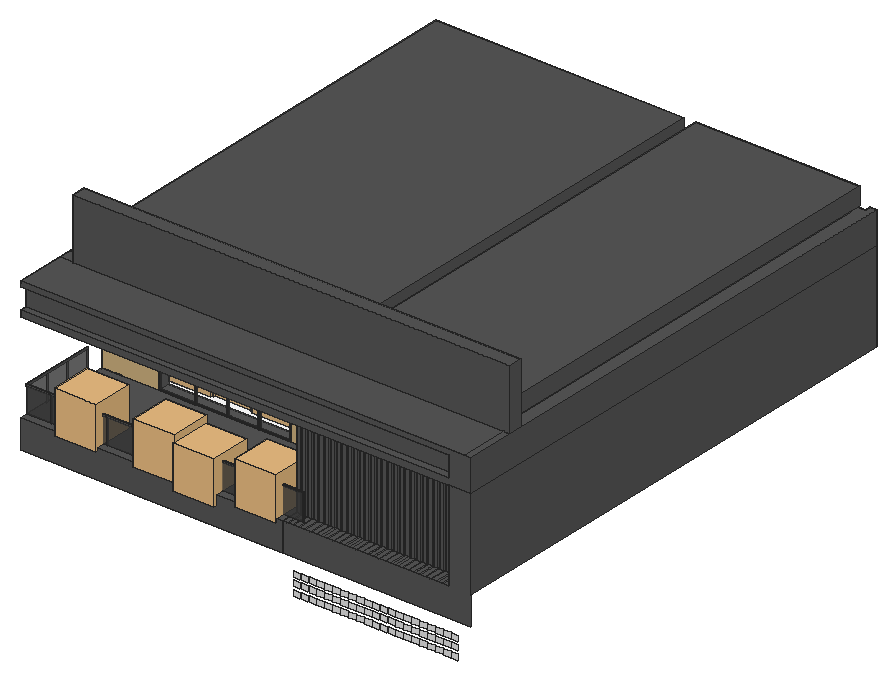
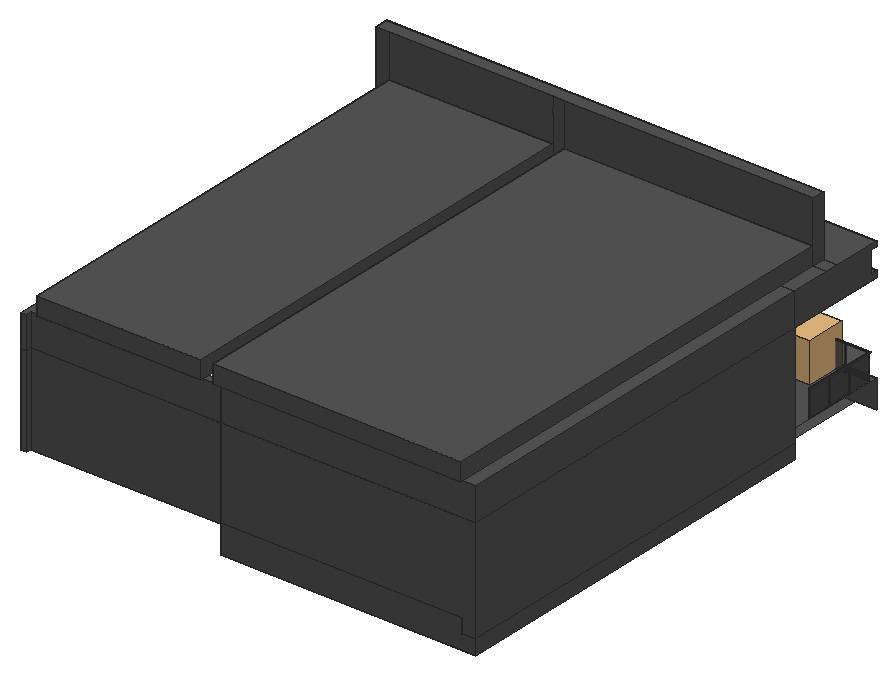
# SketchUp Ruby script. Lengths in inches.
U = 1.inch
M = Sketchup.active_model
def pt(a) = Geom::Point3d.new(a.map { |v| v * U })
def face(e, loops, mat)
  f = e.add_face(loops[0].map { |a| pt(a) })
  loops[1..].each { |l| e.add_face(l.map { |a| pt(a) }).erase! }
  f.material = f.back_material = mat if mat
  f
end
# faces: each face lists its corners as indices into pts; further lists are holes
def faces(e, pts, list, mat = nil) = list.each { |f| face(e, (f[0].is_a?(Array) ? f : [f]).map { |l| l.map { |i| pts[i] } }, mat) }
# xy, xz, yz: faces in a plane at the given z, y or x. An outline is a flat list of corners, or four numbers for a rectangle; further outlines are holes
def ring(l) = l.size == 4 ? [[l[0], l[1]], [l[2], l[1]], [l[2], l[3]], [l[0], l[3]]] : l.each_slice(2).to_a
def flat(e, list, mat, &to3) = list.each { |f| face(e, (f[0].is_a?(Array) ? f : [f]).map { |l| ring(l).map { |u, v| to3.(u, v) } }, mat) }
def xy(e, z, list, mat = nil) = flat(e, list, mat) { |x, y| [x, y, z] }
def xz(e, y, list, mat = nil) = flat(e, list, mat) { |x, z| [x, y, z] }
def yz(e, x, list, mat = nil) = flat(e, list, mat) { |y, z| [x, y, z] }
def lines(e, pts, list) = list.each { |a, b| e.add_line(pt(pts[a]), pt(pts[b])) }
# prism: a flat outline (further loops are holes) pulled along v
def prism(e, loops, v, mat = nil)
  f = face(e, loops, mat); d = Geom::Vector3d.new(v.map { |x| x * U })
  f.pushpull(f.normal.samedirection?(d) ? d.length : -d.length)
end
def box(e, o, s, mat = nil) = prism(e, [[o, [o[0] + s[0], o[1], o[2]], [o[0] + s[0], o[1] + s[1], o[2]], [o[0], o[1] + s[1], o[2]]]], [0, 0, s[2]], mat)
def at(x, y, z, deg = 0) = Geom::Transformation.translation(pt([x, y, z])) * Geom::Transformation.rotation(ORIGIN, Z_AXIS, deg.degrees)
def axes(o, x, y, z) = Geom::Transformation.new([*x, 0, *y, 0, *z, 0, *pt(o).to_a, 1])
def part(name) = M.definitions.add(name)
# library, detail: a bought-in or finely detailed component or shape, given as its bounding box
def library(name, o, s) = part(name).tap { |d| box(d.entities, o, s) }
def detail(e, o, s) = box(e.add_group.entities, o, s)
def put(e, d, t, mat = nil) = e.add_instance(d, t).tap { |i| i.material = mat if mat }
def group(e, t, mat = nil) = e.add_group.tap { |g| g.transformation = t; g.material = mat if mat }.entities
root = M.entities
M.materials.add("Glazing").color = [128, 128, 128]
M.materials["Glazing"].alpha = 0.05
M.materials.add("Powdercoating").color = [41, 44, 40]
M.materials.add("[0135_DarkGray]").color = [81, 81, 81]
M.materials.add("[Color M06]").color = [86, 86, 86]
M.materials.add("[Polished Concrete Old]").color = [229, 229, 229]
M.materials.add("[Translucent Glass Safety]").color = [204, 235, 244]
M.materials["[Translucent Glass Safety]"].alpha = 0.5
M.materials.add("[Translucent_Glass_Gray]").color = [63, 63, 63]
M.materials["[Translucent_Glass_Gray]"].alpha = 0.54
M.materials.add("[Wood Floor Light]").color = [204, 176, 127]
c1 = library("Pot+Plant",[-20.81,-17.08,-0.03],[39.86,39.43,41.33])
c2 = part("Group\#15")
xy(c2.entities,0,[[0,-55.94,0.71,45.94]])
xy(c2.entities,0.2,[[0,-55.94,0.47,45.94],[0.47,45.94,0.71,46.42]])
xy(c2.entities,2.36,[[0.47,-55.94,0.71,46.42]])
xz(c2.entities,-55.94,[[0,0,0.71,0,0.71,2.36,0.47,2.36,0.47,0.2,0,0.2]])
xz(c2.entities,45.94,[[0,0,0.71,0.2]])
xz(c2.entities,46.42,[[0.47,0.2,0.71,2.36]])
yz(c2.entities,0,[[-55.94,0,45.94,0.2]])
yz(c2.entities,0.47,[[-55.94,0.2,46.42,2.36]])
yz(c2.entities,0.71,[[-55.94,0,45.94,0,45.94,0.2,46.42,0.2,46.42,2.36,-55.94,2.36]])
c3 = part("Group\#7")
xy(c3.entities,0,[[0,-59.09,0.71,45.94]])
xy(c3.entities,0.2,[[0,-59.09,0.47,45.94],[0.47,45.94,0.71,46.42]])
xy(c3.entities,2.36,[[0.47,-59.09,0.71,46.42]])
xz(c3.entities,-59.09,[[0,0,0.71,0,0.71,2.36,0.47,2.36,0.47,0.2,0,0.2]])
xz(c3.entities,45.94,[[0,0,0.71,0.2]])
xz(c3.entities,46.42,[[0.47,0.2,0.71,2.36]])
yz(c3.entities,0,[[-59.09,0,45.94,0.2]])
yz(c3.entities,0.47,[[-59.09,0.2,46.42,2.36]])
yz(c3.entities,0.71,[[-59.09,0,45.94,0,45.94,0.2,46.42,0.2,46.42,2.36,-59.09,2.36]])
c4 = part("Group\#16")
prism(c4.entities,[[[0.47,-56.18,0.2],[0,-56.18,0.2],[0,-56.18,0],[0.71,-56.18,0],[0.71,-56.18,2.36],[0.47,-56.18,2.36]]],[0,28.68,0])
c5 = part("Group\#10")
box(c5.entities,[-0.73,0,0],[27.99,0.55,102.05])
c6 = part("Group\#18")
xy(c6.entities,0,[[0.47,-56.18,0.47,-55.47,0,-55.47,0,-28.21,1.18,-28.21,1.18,-56.18]])
xy(c6.entities,0.2,[[0.71,-56.18,1.18,-28.21],[0,-55.47,0.47,-28.21],[0.47,-28.21,0.71,-27.74]])
xy(c6.entities,2.36,[[0.47,-56.18,0.71,-27.74]])
xz(c6.entities,-56.18,[[0.47,0,1.18,0,1.18,0.2,0.71,0.2,0.71,2.36,0.47,2.36]])
xz(c6.entities,-55.47,[[0,0,0.47,0.2]])
xz(c6.entities,-28.21,[[0,0,1.18,0.2]])
xz(c6.entities,-27.74,[[0.47,0.2,0.71,2.36]])
yz(c6.entities,0,[[-55.47,0,-28.21,0.2]])
yz(c6.entities,0.47,[[-56.18,0,-55.47,0.2],[-56.18,0.2,-27.74,2.36]])
yz(c6.entities,0.71,[[-56.18,0.2,-27.74,2.36]])
yz(c6.entities,1.18,[[-56.18,0,-28.21,0.2]])
c7 = part("Group\#34")
xy(c7.entities,0,[[-20.45,0,7.76,1.22]])
xy(c7.entities,0.06,[[-20.39,0.06,7.7,1.22]])
xy(c7.entities,0.47,[[-19.98,0,7.28,0.06]])
xy(c7.entities,101.89,[[-19.98,0,7.28,0.06]])
xy(c7.entities,102.3,[[-20.39,0.06,7.7,1.22]])
xy(c7.entities,102.36,[[-20.45,0,7.76,1.22]])
xz(c7.entities,0,[[[-20.45,0,7.76,102.36],[-19.98,0.47,7.28,101.89]]])
xz(c7.entities,0.06,[[[-20.39,0.06,7.7,102.3],[-19.98,0.47,7.28,101.89]]])
xz(c7.entities,1.22,[[[-20.45,0,7.76,102.36],[-20.39,0.06,7.7,102.3]]])
yz(c7.entities,-20.45,[[0,0,1.22,102.36]])
yz(c7.entities,-20.39,[[0.06,0.06,1.22,102.3]])
yz(c7.entities,-19.98,[[0,0.47,0.06,101.89]])
yz(c7.entities,7.28,[[0,0.47,0.06,101.89]])
yz(c7.entities,7.7,[[0.06,0.06,1.22,102.3]])
yz(c7.entities,7.76,[[0,0,1.22,102.36]])
c8 = part("Group\#6")
put(c8.entities,c2,axes([27.97,0,7.875],[1,0,0],[0,0,-1],[0,1,0]),"Powdercoating")
put(c8.entities,c3,axes([0.71,0,6.8],[-1,0,0],[0,0,-0.97687],[0,1,0]),"Powdercoating")
put(c8.entities,c4,axes([-27.5,0,-38.07],[0,0,-1],[-1,0,0],[0,1,0]),"Powdercoating")
put(c8.entities,c5,at(1.12,0.35,-38.39),"Glazing")
put(c8.entities,c6,axes([-27.5,0,63.35],[0,0,1],[-1,0,0],[0,1,0]),"Powdercoating")
put(c8.entities,c7,at(20.6875,1.0625,-38.54),"Powdercoating")
c9 = part("Sliding door panels")
put(c9.entities,c8,at(-1.18,4.5,38.86))
g1 = group(c9.entities,at(84.74,4.5,38.86))
put(g1,c2,axes([-27.97,0,7.875],[-1,0,0],[0,0,-1],[0,1,0]),"Powdercoating")
put(g1,c3,axes([-0.71,0,6.8],[1,0,0],[0,0,-0.97687],[0,1,0]),"Powdercoating")
put(g1,c4,axes([27.5,0,-38.07],[0,0,-1],[1,0,0],[0,1,0]),"Powdercoating")
put(g1,c5,axes([-1.12,0.35,-38.39],[-1,0,0],[0,1,0],[0,0,1]),"Glazing")
put(g1,c6,axes([27.5,0,63.35],[0,0,1],[1,0,0],[0,1,0]),"Powdercoating")
put(g1,c7,axes([-20.6875,1.0625,-38.54],[-1,0,0],[0,1,0],[0,0,1]),"Powdercoating")
g2 = group(c9.entities,at(56.0625,4.5,38.86))
put(g2,c2,axes([-27.97,0,7.875],[-1,0,0],[0,0,-1],[0,1,0]),"Powdercoating")
put(g2,c4,axes([27.5,0,-38.07],[0,0,-1],[1,0,0],[0,1,0]),"Powdercoating")
put(g2,c5,axes([-1.12,0.35,-38.39],[-1,0,0],[0,1,0],[0,0,1]),"Glazing")
put(g2,c6,axes([27.5,0,63.35],[0,0,1],[1,0,0],[0,1,0]),"Powdercoating")
put(g2,c7,axes([-20.6875,1.0625,-38.54],[-1,0,0],[0,1,0],[0,0,1]),"Powdercoating")
g3 = group(g2,at(-0.71,0,6.8),"Powdercoating")
xy(g3,-45.34,[[0.47,0.2,0.71,2.36]])
xy(g3,-44.88,[[0,0,0.71,0.2]])
xy(g3,57.73,[[0,0,0.71,0,0.71,2.36,0.47,2.36,0.47,0.2,0,0.2]])
xz(g3,0,[[0,-44.88,0.71,57.73]])
xz(g3,0.2,[[0.47,-45.34,0.71,-44.88],[0,-44.88,0.47,57.73]])
xz(g3,2.36,[[0.47,-45.34,0.71,57.73]])
yz(g3,0,[[0,-44.88,0.2,57.73]])
yz(g3,0.47,[[0.2,-45.34,2.36,57.73]])
yz(g3,0.71,[[0.2,-45.34,2.36,-45.34,2.36,57.73,0,57.73,0,-44.88,0.2,-44.88]])
put(c9.entities,c8,axes([-33.94,4.5,38.86],[1.14218,0,0],[0,1,0],[0,0,1]))
c10 = part("sliding door")
put(c10.entities,c9,at(0,-4.5,-0.08))
c11 = part("Group\#81")
box(c11.entities,[0,0,0],[0.79,39.37,35.43],"[Translucent_Glass_Gray]")
c12 = part("Group\#82")
box(c12.entities,[0,0,0],[0.59,1.57,34.25])
c13 = part("Group\#85")
g4 = group(c13.entities,at(0.55,0.5,0))
put(g4,c11,axes([293.06,0,0],[0,0.84,0],[-0.92977,0,0],[0,0,1]),"[Translucent Glass Safety]")
g5 = group(g4,at(0,33.57,0),"[Translucent Glass Safety]")
box(g5,[0,0,0],[0.73,33.07,35.43],"[Translucent_Glass_Gray]")
put(g4,c11,axes([218.38,0,0],[0,0.84,0],[-0.92977,0,0],[0,0,1]),"[Translucent Glass Safety]")
put(g4,c11,axes([367.73,0,0],[0,0.84,0],[-0.92977,0,0],[0,0,1]),"[Translucent Glass Safety]")
g6 = group(g4,at(31.69,0,0),"[Translucent Glass Safety]")
box(g6,[-30.96,0,0],[30.96,0.66,35.43],"[Translucent_Glass_Gray]")
put(g4,c11,axes([255.72,0,0],[0,0.84,0],[-0.92977,0,0],[0,0,1]),"[Translucent Glass Safety]")
g7 = group(g4,at(181.04,0,0),"[Translucent Glass Safety]")
box(g7,[-36.61,0,0],[36.61,0.66,35.43],"[Translucent_Glass_Gray]")
g8 = group(g4,at(0,0.66,0),"[Translucent Glass Safety]")
box(g8,[0,0,0],[0.73,32.24,35.43],"[Translucent_Glass_Gray]")
g9 = group(g4,at(143.71,0,0),"[Translucent Glass Safety]")
box(g9,[-36.61,0,0],[36.61,0.66,35.43],"[Translucent_Glass_Gray]")
g10 = group(g4,at(69.03,0,0),"[Translucent Glass Safety]")
box(g10,[-36.61,0,0],[36.61,0.66,35.43],"[Translucent_Glass_Gray]")
g11 = group(g4,at(0,67.3,0),"[Translucent Glass Safety]")
box(g11,[0,0,0],[0.73,33.07,35.43],"[Translucent_Glass_Gray]")
put(g4,c12,axes([107.44,0.66,0],[0,1,0],[-0.92977,0,0],[0,0,1]),"[0135_DarkGray]")
put(g4,c12,axes([144.78,0.66,0],[0,1,0],[-0.92977,0,0],[0,0,1]),"[0135_DarkGray]")
put(g4,c12,axes([182.11,0.66,0],[0,1,0],[-0.92977,0,0],[0,0,1]),"[0135_DarkGray]")
put(g4,c12,axes([256.79,0.66,0],[0,1,0],[-0.92977,0,0],[0,0,1]),"[0135_DarkGray]")
put(g4,c12,axes([368.14,0.66,0],[0,1,0],[-0.92977,0,0],[0,0,1]),"[0135_DarkGray]")
put(g4,c12,axes([0.73,98.83,0],[0.92977,0,0],[0,1,0],[0,0,1]),"[0135_DarkGray]")
put(g4,c12,axes([331.46,0.66,0],[0,1,0],[-0.92977,0,0],[0,0,1]),"[0135_DarkGray]")
g12 = group(g4,at(106.37,0,0),"[Translucent Glass Safety]")
box(g12,[-36.61,0,0],[36.61,0.66,35.43],"[Translucent_Glass_Gray]")
put(g4,c11,axes([330.39,0,0],[0,0.84,0],[-0.92977,0,0],[0,0,1]),"[Translucent Glass Safety]")
put(g4,c12,axes([294.125,0.66,0],[0,1,0],[-0.92977,0,0],[0,0,1]),"[0135_DarkGray]")
put(g4,c12,axes([0.73,66.04,0],[0.92977,0,0],[0,1,0],[0,0,1]),"[0135_DarkGray]")
put(g4,c12,axes([0.73,32.31,0],[0.92977,0,0],[0,1,0],[0,0,1]),"[0135_DarkGray]")
put(g4,c12,axes([32.76,0.66,0],[0,1,0],[-0.92977,0,0],[0,0,1]),"[0135_DarkGray]")
put(g4,c12,axes([70.1,0.66,0],[0,1,0],[-0.92977,0,0],[0,0,1]),"[0135_DarkGray]")
put(g4,c12,axes([219.45,0.66,0],[0,1,0],[-0.92977,0,0],[0,0,1]),"[0135_DarkGray]")
g13 = group(c13.entities,at(0,0,34.25))
xy(g13,0,[[0,0,0,100.87,0.55,100.87,0.55,0.5,362.73,0.5,362.73,0],[362.73,0,369.35,0.5],[368.19,0.5,368.6875,1.16],[1.28,1.16,1.28,100.87,1.83,100.87,1.83,1.65,362.73,1.65,362.73,1.16],[362.73,1.16,368.19,1.65]],"[0135_DarkGray]")
xy(g13,1.18,[[368.19,0,368.6875,0.5],[368.6875,0,369.35,0.5],[0.55,0.5,0.55,100.87,1.28,100.87,1.28,1.16,362.73,1.16,362.73,0.5],[368.6875,0.5,369.35,1.16]],"[0135_DarkGray]")
xy(g13,1.97,[[0,0,362.73,0,362.73,1.65,1.83,1.65,1.83,100.87,0,100.87],[362.73,0,368.19,1.65]],"[0135_DarkGray]")
xz(g13,0,[[0,0,362.73,1.97],[362.73,0,369.35,0,369.35,1.18,368.19,1.18,368.19,1.97,362.73,1.97]],"[0135_DarkGray]")
xz(g13,0.5,[[0.55,0,1.28,1.18],[1.28,0,362.73,1.18],[362.73,0,368.19,1.18],[368.19,0,368.6875,1.18],[368.6875,0,369.35,1.18]],"[0135_DarkGray]")
xz(g13,1.16,[[1.28,0,362.73,1.18],[362.73,0,368.19,1.18]],"[0135_DarkGray]")
xz(g13,1.65,[[1.83,0,362.73,1.97],[362.73,0,368.19,1.97]],"[0135_DarkGray]")
xz(g13,100.87,[[0,0,0,1.97,1.83,1.97,1.83,0,1.28,0,1.28,1.18,0.55,1.18,0.55,0]],"[0135_DarkGray]")
yz(g13,0,[[0,0,100.87,1.97]],"[0135_DarkGray]")
yz(g13,0.55,[[0.5,0,100.87,1.18]],"[0135_DarkGray]")
yz(g13,1.28,[[1.16,0,100.87,1.18]],"[0135_DarkGray]")
yz(g13,1.83,[[1.65,0,100.87,1.97]],"[0135_DarkGray]")
yz(g13,362.73,[[0,0,0,1.97,1.65,1.97,1.65,0,1.16,0,1.16,1.18,0.5,1.18,0.5,0]],"[0135_DarkGray]")
yz(g13,368.19,[[1.16,0,1.65,0,1.65,1.97,0,1.97,0,1.18,1.16,1.18],[0.5,0,1.16,1.18]],"[0135_DarkGray]")
yz(g13,368.6875,[[0.5,0,1.16,1.18]],"[0135_DarkGray]")
yz(g13,369.35,[[0,0,0.5,1.18]],"[0135_DarkGray]")
c14 = library("Group14",[-64.97,9.24,0.31],[138.52,9.93,292.57])
c15 = library("Group16",[86.37,-10.76,76.46],[21.79,14.87,35.97])
c16 = library("Group22",[48.82,-10.91,0.23],[97.72,18.57,293.12])
c17 = library("Group24",[44.03,2.01,0.26],[103.73,11,292.35])
c18 = library("Group27",[-106.21,-10.76,76.46],[21.8,14.87,35.97])
c19 = library("Group35",[-145.81,2.01,0.26],[103.73,11,292.35])
c20 = library("Group33",[-144.59,-10.91,0.23],[97.72,18.57,293.12])
c21 = part("rem")
g14 = group(c21.entities,at(-145.81,-10.91,0.23))
put(g14,c14,at(145.81,10.91,-0.23))
put(g14,c15,at(145.81,10.91,-0.23))
put(g14,c16,at(145.81,10.91,-0.23))
put(g14,c17,at(145.81,10.91,-0.23))
put(g14,c18,at(145.81,10.91,-0.23))
put(g14,c19,at(145.81,10.91,-0.23))
put(g14,c20,at(145.81,10.91,-0.23))
xy(root,521.33,[[72.77,145.99,251.64,161.89]],"[Color M06]")
xy(root,537.58,[[29.53,10.05,45.84,145.99],[45.84,10.05,45.84,145.99,349.9,145.99,349.9,92.58,333.03,92.58,333.03,10.05],[333.03,10.05,349.9,82.9],[333.03,82.9,349.9,92.58],[1.28,145.99,1.28,675.01,340.92,675.01,340.92,665.33,29.53,665.33,29.53,161.89,349.9,161.89,349.9,145.99]],"[Color M06]")
xy(root,557.15,[[1.28,145.99,19.84,675.01]],"[Color M06]")
xy(root,575.27,[[365.22,92.58,582.75,161.89]],"[Color M06]")
xy(root,575.71,[[1.28,10.05,349.9,10.05,349.9,145.99,252.22,145.99,252.22,161.89,76.62,161.89,76.62,145.99,1.28,145.99],[349.9,10.05,355.47,33.18],[355.47,10.05,357.53,82.9],[357.53,10.05,363.1,32.62],[363.1,10.05,365.15,82.9],
  [365.15,10.05,370.72,32.62],[370.72,10.05,372.78,82.9],[372.78,10.05,378.35,32.62],[378.35,10.05,380.4,82.9],[380.4,10.05,385.97,32.62],
  [385.97,10.05,388.03,82.9],[388.03,10.05,393.6,32.62],[393.6,10.05,395.65,82.9],[395.65,10.05,401.22,32.62],[401.22,10.05,403.28,82.9],
  [403.28,10.05,408.85,32.62],[408.85,10.05,410.9,82.9],[410.9,10.05,416.47,32.62],[416.47,10.05,418.53,82.9],[418.53,10.05,424.1,32.62],
  [424.1,10.05,426.15,82.9],[426.15,10.05,431.72,32.62],[431.72,10.05,433.78,82.9],[433.78,10.05,439.35,32.62],[439.35,10.05,441.4,82.9],
  [441.4,10.05,446.97,32.62],[446.97,10.05,449.03,82.9],[449.03,10.05,454.6,32.62],[454.6,10.05,456.65,82.9],[456.65,10.05,462.22,32.62],
  [462.22,10.05,464.28,82.9],[464.28,10.05,469.85,32.62],[469.85,10.05,471.9,82.9],[471.9,10.05,477.47,32.62],[477.47,10.05,479.53,82.9],
  [479.53,10.05,485.1,32.62],[485.1,10.05,487.15,82.9],[487.15,10.05,492.72,32.62],[492.72,10.05,494.78,82.9],[494.78,10.05,500.35,32.62],
  [500.35,10.05,502.4,82.9],[502.4,10.05,507.97,32.62],[507.97,10.05,510.03,82.9],[510.03,10.05,515.6,32.62],[515.6,10.05,517.65,82.9],
  [517.65,10.05,523.22,32.62],[523.22,10.05,525.28,82.9],[525.28,10.05,530.85,32.62],[530.85,10.05,532.9,82.9],[532.9,10.05,538.47,32.62],
  [538.47,10.05,540.53,82.9],[540.53,10.05,546.1,32.62],[546.1,10.05,548.15,82.9],[548.15,10.05,553.72,32.62],[553.72,10.05,555.78,82.9],
  [555.78,10.05,561.35,32.62],[561.35,10.05,563.4,82.9],[563.4,10.05,568.97,32.62],[568.97,10.05,570.33,82.9],[19.84,145.99,19.84,675.01,340.92,675.01,340.92,665.33,29.53,665.33,29.53,161.89,76.62,161.89,76.62,145.99],
  [252.22,145.99,349.9,161.89]],"[Color M06]")
xy(root,684.24,[[76.62,145.99,252.22,161.89]],"[Color M06]")
xy(root,695.71,[[1.28,10.05,1.28,145.99,15.1,145.99,15.1,33.18,345.85,33.18,357.53,33.15,357.53,32.62,363.1,32.62,363.1,33.14,365.15,33.13,365.15,32.62,370.72,32.62,370.72,33.12,372.78,33.11,372.78,32.62,378.35,32.62,378.35,33.1,380.4,33.1,380.4,32.62,385.97,32.62,385.97,33.08,388.03,33.08,388.03,32.62,393.6,32.62,393.6,33.0625,395.65,33.06,395.65,32.62,401.22,32.62,401.22,33.04,403.28,33.04,403.28,32.62,408.85,32.62,408.85,33.02,410.9,33.02,410.9,32.62,416.47,32.62,416.47,33,418.53,33,418.53,32.62,424.1,32.62,424.1,32.99,426.15,32.98,426.15,32.62,431.72,32.62,431.72,32.97,433.78,32.96,433.78,32.62,439.35,32.62,439.35,32.95,441.4,32.94,441.4,32.62,446.97,32.62,446.97,32.93,449.03,32.92,449.03,32.62,454.6,32.62,454.6,32.91,456.65,32.9,456.65,32.62,462.22,32.62,462.22,32.89,464.28,32.88,464.28,32.62,469.85,32.62,469.85,32.87,471.9,32.86,471.9,32.62,477.47,32.62,477.47,32.85,479.53,32.85,479.53,32.62,485.1,32.62,485.1,32.83,487.15,32.83,487.15,32.62,492.72,32.62,492.72,32.8125,494.78,32.81,494.78,32.62,500.35,32.62,500.35,32.79,502.4,32.79,502.4,32.62,507.97,32.62,507.97,32.77,510.03,32.77,510.03,32.62,515.6,32.62,515.6,32.75,517.65,32.75,517.65,32.62,523.22,32.62,523.22,32.74,525.28,32.73,525.28,32.62,530.85,32.62,530.85,32.72,532.9,32.71,532.9,32.62,538.47,32.62,538.47,32.7,540.53,32.69,540.53,32.62,546.1,32.62,546.1,32.68,548.15,32.67,548.15,32.62,553.72,32.62,553.72,32.66,555.78,32.65,555.78,32.62,561.35,32.62,561.35,32.64,563.4,32.63,563.4,32.62,568.97,32.62,568.97,82.9,570.33,82.9,570.33,10.05],[570.33,10.05,570.33,82.9,568.97,82.9,568.97,32.62,563.4,32.63,563.4,82.9,561.35,82.9,561.35,32.64,555.78,32.65,555.78,82.9,553.72,82.9,553.72,32.66,548.15,32.67,548.15,82.9,546.1,82.9,546.1,32.68,540.53,32.69,540.53,82.9,538.47,82.9,538.47,32.7,532.9,32.71,532.9,82.9,530.85,82.9,530.85,32.72,525.28,32.73,525.28,82.9,523.22,82.9,523.22,32.74,517.65,32.75,517.65,82.9,515.6,82.9,515.6,32.75,510.03,32.77,510.03,82.9,507.97,82.9,507.97,32.77,502.4,32.79,502.4,82.9,500.35,82.9,500.35,32.79,494.78,32.81,494.78,82.9,492.72,82.9,492.72,32.8125,487.15,32.83,487.15,82.9,485.1,82.9,485.1,32.83,479.53,32.85,479.53,82.9,477.47,82.9,477.47,32.85,471.9,32.86,471.9,82.9,469.85,82.9,469.85,32.87,464.28,32.88,464.28,82.9,462.22,82.9,462.22,32.89,456.65,32.9,456.65,82.9,454.6,82.9,454.6,32.91,449.03,32.92,449.03,82.9,446.97,82.9,446.97,32.93,441.4,32.94,441.4,82.9,439.35,82.9,439.35,32.95,433.78,32.96,433.78,82.9,431.72,82.9,431.72,32.97,426.15,32.98,426.15,82.9,424.1,82.9,424.1,32.99,418.53,33,418.53,82.9,416.47,82.9,416.47,33,410.9,33.02,410.9,82.9,408.85,82.9,408.85,33.02,403.28,33.04,403.28,82.9,401.22,82.9,401.22,33.04,395.65,33.06,395.65,82.9,393.6,82.9,393.6,33.0625,388.03,33.08,388.03,82.9,385.97,82.9,385.97,33.08,380.4,33.1,380.4,82.9,378.35,82.9,378.35,33.1,372.78,33.11,372.78,82.9,370.72,82.9,370.72,33.12,365.15,33.13,365.15,82.9,363.1,82.9,363.1,33.14,357.53,33.15,357.53,82.9,355.47,82.9,355.47,33.18,349.9,33.18,349.9,161.89,365.22,161.89,365.22,92.58,582.75,92.58,582.75,665.33,340.92,665.33,340.92,675.01,592.4375,675.01,592.4375,683.05,600.47,683.05,600.47,10.05],[357.53,32.62,357.53,33.15,363.1,33.14,363.1,32.62],[365.15,32.62,365.15,33.13,370.72,33.12,370.72,32.62],[372.78,32.62,372.78,33.11,378.35,33.1,378.35,32.62],
  [380.4,32.62,380.4,33.1,385.97,33.08,385.97,32.62],[388.03,32.62,388.03,33.08,393.6,33.0625,393.6,32.62],[395.65,32.62,395.65,33.06,401.22,33.04,401.22,32.62],[403.28,32.62,403.28,33.04,408.85,33.02,408.85,32.62],[410.9,32.62,410.9,33.02,416.47,33,416.47,32.62],
  [418.53,32.62,418.53,33,424.1,32.99,424.1,32.62],[426.15,32.62,426.15,32.98,431.72,32.97,431.72,32.62],[433.78,32.62,433.78,32.96,439.35,32.95,439.35,32.62],[441.4,32.62,441.4,32.94,446.97,32.93,446.97,32.62],[449.03,32.62,449.03,32.92,454.6,32.91,454.6,32.62],
  [456.65,32.62,456.65,32.9,462.22,32.89,462.22,32.62],[464.28,32.62,464.28,32.88,469.85,32.87,469.85,32.62],[471.9,32.62,471.9,32.86,477.47,32.85,477.47,32.62],[479.53,32.62,479.53,32.85,485.1,32.83,485.1,32.62],[487.15,32.62,487.15,32.83,492.72,32.8125,492.72,32.62],
  [494.78,32.62,494.78,32.81,500.35,32.79,500.35,32.62],[502.4,32.62,502.4,32.79,507.97,32.77,507.97,32.62],[510.03,32.62,510.03,32.77,515.6,32.75,515.6,32.62],[517.65,32.62,517.65,32.75,523.22,32.74,523.22,32.62],[525.28,32.62,525.28,32.73,530.85,32.72,530.85,32.62],
  [532.9,32.62,532.9,32.71,538.47,32.7,538.47,32.62],[540.53,32.62,540.53,32.69,546.1,32.68,546.1,32.62],[548.15,32.62,548.15,32.67,553.72,32.66,553.72,32.62],[555.78,32.62,555.78,32.65,561.35,32.64,561.35,32.62],[563.4,32.62,563.4,32.63,568.97,32.62],
  [563.4,32.63,561.35,32.64,561.35,82.9,563.4,82.9],[555.78,32.65,553.72,32.66,553.72,82.9,555.78,82.9],[548.15,32.67,546.1,32.68,546.1,82.9,548.15,82.9],[540.53,32.69,538.47,32.7,538.47,82.9,540.53,82.9],[532.9,32.71,530.85,32.72,530.85,82.9,532.9,82.9],
  [525.28,32.73,523.22,32.74,523.22,82.9,525.28,82.9],[515.6,32.75,517.65,82.9],[507.97,32.77,510.03,82.9],[500.35,32.79,502.4,82.9],[494.78,32.81,492.72,32.8125,492.72,82.9,494.78,82.9],
  [485.1,32.83,487.15,82.9],[477.47,32.85,479.53,82.9],[471.9,32.86,469.85,32.87,469.85,82.9,471.9,82.9],[464.28,32.88,462.22,32.89,462.22,82.9,464.28,82.9],[456.65,32.9,454.6,32.91,454.6,82.9,456.65,82.9],
  [449.03,32.92,446.97,32.93,446.97,82.9,449.03,82.9],[441.4,32.94,439.35,32.95,439.35,82.9,441.4,82.9],[433.78,32.96,431.72,32.97,431.72,82.9,433.78,82.9],[426.15,32.98,424.1,32.99,424.1,82.9,426.15,82.9],[416.47,33,418.53,82.9],
  [408.85,33.02,410.9,82.9],[401.22,33.04,403.28,82.9],[395.65,33.06,393.6,33.0625,393.6,82.9,395.65,82.9],[385.97,33.08,388.03,82.9],[378.35,33.1,380.4,82.9],
  [372.78,33.11,370.72,33.12,370.72,82.9,372.78,82.9],[365.15,33.13,363.1,33.14,363.1,82.9,365.15,82.9],[357.53,33.15,345.85,33.18,355.47,33.18,355.47,82.9,357.53,82.9],[1.28,145.99,1.28,675.01,340.92,675.01,340.92,665.33,29.53,665.33,29.53,161.89,349.9,161.89,349.9,145.99]],"[Color M06]")
xy(root,695.71,[[15.1,33.18,349.9,145.99]],"[Wood Floor Light]")
xy(root,704.31,[[1.28,10.05,570.4,19.67]],"[Color M06]")
xy(root,732.18,[[1.28,10.05,570.4,19.67]],"[Color M06]")
xy(root,739.02,[[1.28,10.05,592.4375,74.86],[592.4375,10.05,600.47,74.86],[1.28,74.86,19.84,92.58],[19.84,74.86,600.47,92.58],[1.28,92.58,19.84,145.99],
  [19.84,92.58,19.84,675.01,340.92,675.01,340.92,665.33,29.53,665.33,29.53,161.89,349.9,161.89,349.9,92.58],[349.9,92.58,365.22,161.89],[365.22,92.58,582.75,665.33],[582.75,92.58,600.47,92.58,600.47,683.05,592.4375,683.05,592.4375,675.01,582.75,675.01],[1.28,145.99,19.84,675.01],
  [29.53,161.89,349.9,665.33],[340.92,665.33,349.9,675.01],[349.9,665.33,365.22,675.01],[365.22,665.33,582.75,675.01],[19.84,675.01,349.9,677.15],
  [365.22,675.01,582.75,677.15]],"[Color M06]")
xy(root,762.9,[[19.84,92.58,349.9,677.15],[365.22,92.58,582.75,677.15]],"[Color M06]")
xy(root,819.77,[[19.84,74.86,600.47,92.58]],"[Color M06]")
xz(root,10.05,[[1.28,537.58,349.9,575.71],[349.9,537.58,600.47,537.58,600.47,695.71,570.33,695.71,570.33,575.71,349.9,575.71],[1.28,695.71,600.47,695.71,600.47,739.02,1.28,739.02,1.28,732.18,570.4,732.18,570.4,704.31,1.28,704.31]],"[Color M06]")
xz(root,10.05,[[364.36,491.43,373.36,498.75],[374.86,491.43,383.86,498.75],[385.36,491.43,394.36,498.75],[395.86,491.43,404.86,498.75],[406.36,491.43,415.36,498.75],
  [416.86,491.43,425.86,498.75],[427.36,491.43,436.36,498.75],[437.86,491.43,446.86,498.75],[448.36,491.43,457.36,498.75],[458.86,491.43,467.86,498.75],
  [469.36,491.43,478.36,498.75],[479.86,491.43,488.86,498.75],[490.36,491.43,499.36,498.75],[500.86,491.43,509.86,498.75],[511.36,491.43,520.36,498.75],
  [521.86,491.43,530.86,498.75],[532.36,491.43,541.36,498.75],[542.86,491.43,551.86,498.75],[553.36,491.43,562.36,498.75],[563.86,491.43,572.86,498.75],
  [574.36,491.43,583.36,498.75],[364.36,503,373.36,510.31],[374.86,503,383.86,510.31],[385.36,503,394.36,510.31],[395.86,503,404.86,510.31],
  [406.36,503,415.36,510.31],[416.86,503,425.86,510.31],[427.36,503,436.36,510.31],[437.86,503,446.86,510.31],[448.36,503,457.36,510.31],
  [458.86,503,467.86,510.31],[469.36,503,478.36,510.31],[479.86,503,488.86,510.31],[490.36,503,499.36,510.31],[500.86,503,509.86,510.31],
  [511.36,503,520.36,510.31],[521.86,503,530.86,510.31],[532.36,503,541.36,510.31],[542.86,503,551.86,510.31],[553.36,503,562.36,510.31],
  [563.86,503,572.86,510.31],[574.36,503,583.36,510.31],[364.36,513.93,373.36,521.25],[374.86,513.93,383.86,521.25],[385.36,513.93,394.36,521.25],
  [395.86,513.93,404.86,521.25],[406.36,513.93,415.36,521.25],[416.86,513.93,425.86,521.25],[427.36,513.93,436.36,521.25],[437.86,513.93,446.86,521.25],
  [448.36,513.93,457.36,521.25],[458.86,513.93,467.86,521.25],[469.36,513.93,478.36,521.25],[479.86,513.93,488.86,521.25],[490.36,513.93,499.36,521.25],
  [500.86,513.93,509.86,521.25],[511.36,513.93,520.36,521.25],[521.86,513.93,530.86,521.25],[532.36,513.93,541.36,521.25],[542.86,513.93,551.86,521.25],
  [553.36,513.93,562.36,521.25],[563.86,513.93,572.86,521.25],[574.36,513.93,583.36,521.25]],"[Polished Concrete Old]")
xz(root,19.67,[[1.28,704.31,570.4,732.18]],"[Color M06]")
xz(root,32.62,[[357.53,575.71,363.1,695.71],[365.15,575.71,370.72,695.71],[372.78,575.71,378.35,695.71],[380.4,575.71,385.97,695.71],[388.03,575.71,393.6,695.71],
  [395.65,575.71,401.22,695.71],[403.28,575.71,408.85,695.71],[410.9,575.71,416.47,695.71],[418.53,575.71,424.1,695.71],[426.15,575.71,431.72,695.71],
  [433.78,575.71,439.35,695.71],[441.4,575.71,446.97,695.71],[449.03,575.71,454.6,695.71],[456.65,575.71,462.22,695.71],[464.28,575.71,469.85,695.71],
  [471.9,575.71,477.47,695.71],[479.53,575.71,485.1,695.71],[487.15,575.71,492.72,695.71],[494.78,575.71,500.35,695.71],[502.4,575.71,507.97,695.71],
  [510.03,575.71,515.6,695.71],[517.65,575.71,523.22,695.71],[525.28,575.71,530.85,695.71],[532.9,575.71,538.47,695.71],[540.53,575.71,546.1,695.71],
  [548.15,575.71,553.72,695.71],[555.78,575.71,561.35,695.71],[563.4,575.71,568.97,695.71]],"[Color M06]")
xz(root,33.18,[[349.9,575.71,355.47,695.71]],"[Color M06]")
xz(root,74.86,[[19.84,739.02,600.47,819.77]],"[Color M06]")
xz(root,82.9,[[355.47,575.71,357.53,695.71],[363.1,575.71,365.15,695.71],[370.72,575.71,372.78,695.71],[378.35,575.71,380.4,695.71],[385.97,575.71,388.03,695.71],
  [393.6,575.71,395.65,695.71],[401.22,575.71,403.28,695.71],[408.85,575.71,410.9,695.71],[416.47,575.71,418.53,695.71],[424.1,575.71,426.15,695.71],
  [431.72,575.71,433.78,695.71],[439.35,575.71,441.4,695.71],[446.97,575.71,449.03,695.71],[454.6,575.71,456.65,695.71],[462.22,575.71,464.28,695.71],
  [469.85,575.71,471.9,695.71],[477.47,575.71,479.53,695.71],[485.1,575.71,487.15,695.71],[492.72,575.71,494.78,695.71],[500.35,575.71,502.4,695.71],
  [507.97,575.71,510.03,695.71],[515.6,575.71,517.65,695.71],[523.22,575.71,525.28,695.71],[530.85,575.71,532.9,695.71],[538.47,575.71,540.53,695.71],
  [546.1,575.71,548.15,695.71],[553.72,575.71,555.78,695.71],[561.35,575.71,563.4,695.71],[568.97,575.71,570.33,695.71]],"[Color M06]")
xz(root,92.58,[[365.22,575.27,582.75,695.71],[365.22,695.71,582.75,739.02],[19.84,739.02,349.9,762.9],[349.9,739.02,365.22,819.77],[365.22,739.02,582.75,762.9],
  [582.75,739.02,600.47,819.77],[19.84,762.9,349.9,819.77],[365.22,762.9,582.75,819.77]],"[Color M06]")
xz(root,145.99,[[1.28,537.58,29.53,537.58,29.53,575.71,19.84,575.71,19.84,557.15,1.28,557.15],[1.28,557.15,19.84,575.71]],"[Color M06]")
xz(root,145.99,[[1.28,575.71,76.62,575.71,76.62,684.24,252.22,684.24,252.22,575.71,349.9,575.71,349.9,695.71,1.28,695.71]],"[Wood Floor Light]")
xz(root,161.89,[[29.53,537.58,349.9,575.71],[349.9,575.27,365.22,695.71],[29.53,575.71,29.53,695.71,349.9,695.71,349.9,575.71,252.22,575.71,252.22,684.24,76.62,684.24,76.62,575.71],[29.53,695.71,349.9,739.02],[349.9,695.71,365.22,739.02]],"[Color M06]")
xz(root,665.33,[[29.53,537.58,340.92,575.71],[340.92,575.27,582.75,695.71],[29.53,575.71,340.92,695.71],[29.53,695.71,340.92,739.02],[340.92,695.71,582.75,739.02]],"[Color M06]")
xz(root,675.01,[[1.28,537.58,1.28,557.15,19.84,557.15,19.84,575.71,340.92,575.71,340.92,537.58],[1.28,557.15,1.28,695.71,340.92,695.71,340.92,575.71,19.84,575.71,19.84,557.15],[340.92,575.27,592.4375,695.71],[1.28,695.71,340.92,739.02],[340.92,695.71,592.4375,739.02]],"[Color M06]")
xz(root,677.15,[[19.84,739.02,349.9,762.9],[365.22,739.02,582.75,762.9]],"[Color M06]")
xz(root,683.05,[[592.4375,575.27,600.47,695.71],[592.4375,695.71,600.47,739.02]],"[Color M06]")
yz(root,1.28,[[145.99,537.58,675.01,557.15],[145.99,557.15,675.01,695.71],[10.05,695.71,10.05,704.31,19.67,704.31,19.67,732.18,10.05,732.18,10.05,739.02,145.99,739.02,145.99,695.71],[145.99,695.71,675.01,739.02]],"[Color M06]")
yz(root,19.84,[[145.99,557.15,675.01,575.71],[74.86,739.02,92.58,819.77],[92.58,739.02,677.15,762.9]],"[Color M06]")
yz(root,29.53,[[161.89,537.58,665.33,575.71],[161.89,575.71,665.33,695.71],[161.89,695.71,665.33,739.02]],"[Color M06]")
yz(root,76.62,[[145.99,575.71,161.89,684.24]],"[Color M06]")
yz(root,252.22,[[145.99,575.71,161.89,684.24]],"[Color M06]")
yz(root,340.92,[[665.33,537.58,675.01,575.27],[665.33,575.27,675.01,575.71],[665.33,575.71,675.01,695.71],[665.33,695.71,675.01,739.02]],"[Color M06]")
yz(root,349.9,[[10.05,537.58,161.89,575.27],[10.05,575.27,161.89,575.71],[33.18,575.71,92.58,695.71],[92.58,575.71,145.99,695.71],[145.99,575.71,161.89,695.71],
  [92.58,739.02,677.15,762.9]],"[Color M06]")
yz(root,355.47,[[33.18,575.71,82.9,695.71]],"[Color M06]")
yz(root,357.53,[[32.62,575.71,82.9,695.71]],"[Color M06]")
yz(root,363.1,[[32.62,575.71,82.9,695.71]],"[Color M06]")
yz(root,365.15,[[32.62,575.71,82.9,695.71]],"[Color M06]")
yz(root,365.22,[[92.58,575.27,161.89,695.71],[92.58,695.71,161.89,739.02],[92.58,739.02,677.15,762.9]],"[Color M06]")
yz(root,370.72,[[32.62,575.71,82.9,695.71]],"[Color M06]")
yz(root,372.78,[[32.62,575.71,82.9,695.71]],"[Color M06]")
yz(root,378.35,[[32.62,575.71,82.9,695.71]],"[Color M06]")
yz(root,380.4,[[32.62,575.71,82.9,695.71]],"[Color M06]")
yz(root,385.97,[[32.62,575.71,82.9,695.71]],"[Color M06]")
yz(root,388.03,[[32.62,575.71,82.9,695.71]],"[Color M06]")
yz(root,393.6,[[32.62,575.71,82.9,695.71]],"[Color M06]")
yz(root,395.65,[[32.62,575.71,82.9,695.71]],"[Color M06]")
yz(root,401.22,[[32.62,575.71,82.9,695.71]],"[Color M06]")
yz(root,403.28,[[32.62,575.71,82.9,695.71]],"[Color M06]")
yz(root,408.85,[[32.62,575.71,82.9,695.71]],"[Color M06]")
yz(root,410.9,[[32.62,575.71,82.9,695.71]],"[Color M06]")
yz(root,416.47,[[32.62,575.71,82.9,695.71]],"[Color M06]")
yz(root,418.53,[[32.62,575.71,82.9,695.71]],"[Color M06]")
yz(root,424.1,[[32.62,575.71,82.9,695.71]],"[Color M06]")
yz(root,426.15,[[32.62,575.71,82.9,695.71]],"[Color M06]")
yz(root,431.72,[[32.62,575.71,82.9,695.71]],"[Color M06]")
yz(root,433.78,[[32.62,575.71,82.9,695.71]],"[Color M06]")
yz(root,439.35,[[32.62,575.71,82.9,695.71]],"[Color M06]")
yz(root,441.4,[[32.62,575.71,82.9,695.71]],"[Color M06]")
yz(root,446.97,[[32.62,575.71,82.9,695.71]],"[Color M06]")
yz(root,449.03,[[32.62,575.71,82.9,695.71]],"[Color M06]")
yz(root,454.6,[[32.62,575.71,82.9,695.71]],"[Color M06]")
yz(root,456.65,[[32.62,575.71,82.9,695.71]],"[Color M06]")
yz(root,462.22,[[32.62,575.71,82.9,695.71]],"[Color M06]")
yz(root,464.28,[[32.62,575.71,82.9,695.71]],"[Color M06]")
yz(root,469.85,[[32.62,575.71,82.9,695.71]],"[Color M06]")
yz(root,471.9,[[32.62,575.71,82.9,695.71]],"[Color M06]")
yz(root,477.47,[[32.62,575.71,82.9,695.71]],"[Color M06]")
yz(root,479.53,[[32.62,575.71,82.9,695.71]],"[Color M06]")
yz(root,485.1,[[32.62,575.71,82.9,695.71]],"[Color M06]")
yz(root,487.15,[[32.62,575.71,82.9,695.71]],"[Color M06]")
yz(root,492.72,[[32.62,575.71,82.9,695.71]],"[Color M06]")
yz(root,494.78,[[32.62,575.71,82.9,695.71]],"[Color M06]")
yz(root,500.35,[[32.62,575.71,82.9,695.71]],"[Color M06]")
yz(root,502.4,[[32.62,575.71,82.9,695.71]],"[Color M06]")
yz(root,507.97,[[32.62,575.71,82.9,695.71]],"[Color M06]")
yz(root,510.03,[[32.62,575.71,82.9,695.71]],"[Color M06]")
yz(root,515.6,[[32.62,575.71,82.9,695.71]],"[Color M06]")
yz(root,517.65,[[32.62,575.71,82.9,695.71]],"[Color M06]")
yz(root,523.22,[[32.62,575.71,82.9,695.71]],"[Color M06]")
yz(root,525.28,[[32.62,575.71,82.9,695.71]],"[Color M06]")
yz(root,530.85,[[32.62,575.71,82.9,695.71]],"[Color M06]")
yz(root,532.9,[[32.62,575.71,82.9,695.71]],"[Color M06]")
yz(root,538.47,[[32.62,575.71,82.9,695.71]],"[Color M06]")
yz(root,540.53,[[32.62,575.71,82.9,695.71]],"[Color M06]")
yz(root,546.1,[[32.62,575.71,82.9,695.71]],"[Color M06]")
yz(root,548.15,[[32.62,575.71,82.9,695.71]],"[Color M06]")
yz(root,553.72,[[32.62,575.71,82.9,695.71]],"[Color M06]")
yz(root,555.78,[[32.62,575.71,82.9,695.71]],"[Color M06]")
yz(root,561.35,[[32.62,575.71,82.9,695.71]],"[Color M06]")
yz(root,563.4,[[32.62,575.71,82.9,695.71]],"[Color M06]")
yz(root,568.97,[[32.62,575.71,82.9,695.71]],"[Color M06]")
yz(root,570.33,[[10.05,575.71,82.9,695.71]],"[Color M06]")
yz(root,570.4,[[10.05,704.31,19.67,732.18]],"[Color M06]")
yz(root,582.75,[[92.58,575.27,665.33,695.71],[92.58,695.71,665.33,739.02],[92.58,739.02,677.15,762.9]],"[Color M06]")
yz(root,592.4375,[[675.01,575.27,683.05,695.71],[675.01,695.71,683.05,739.02]],"[Color M06]")
yz(root,600.47,[[10.05,575.27,683.05,695.71],[10.05,695.71,683.05,739.02],[74.86,739.02,92.58,819.77]],"[Color M06]")
put(root,c1,axes([234.76,30.64,562.52],[1.38,0,0],[0,1.38,0],[0,0,1.38]))
put(root,c1,axes([76.02,32.9375,570.625],[1.38,0,0],[0,1.38,0],[0,0,1.38]))
put(root,c1,axes([180.21,32.9375,570.625],[1.38,0,0],[0,1.38,0],[0,0,1.38]))
put(root,c1,axes([315.09,32.9375,570.625],[1.38,0,0],[0,1.38,0],[0,0,1.38]))
put(root,c10,axes([126.83,145.99,575.71],[1.47956,0,0],[0,1,0],[0,0,1.05053]),"[Color M06]")
put(root,c13,axes([0.82,19.87,575.71],[0.99859,0,0],[0,1,0],[0,0,1]),"[Color M06]")
put(root,c21,axes([159.4375,163.96,580.45],[0.568,0,0],[0,0.19,0],[0,0,0.35379]),"[Color M06]")
